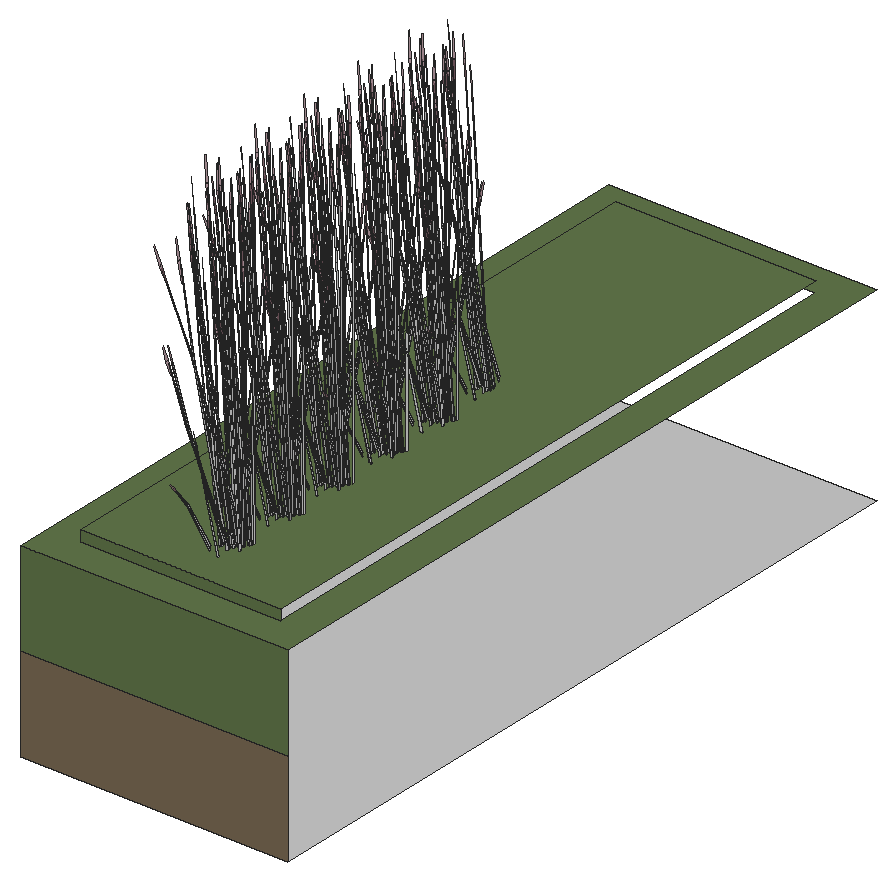
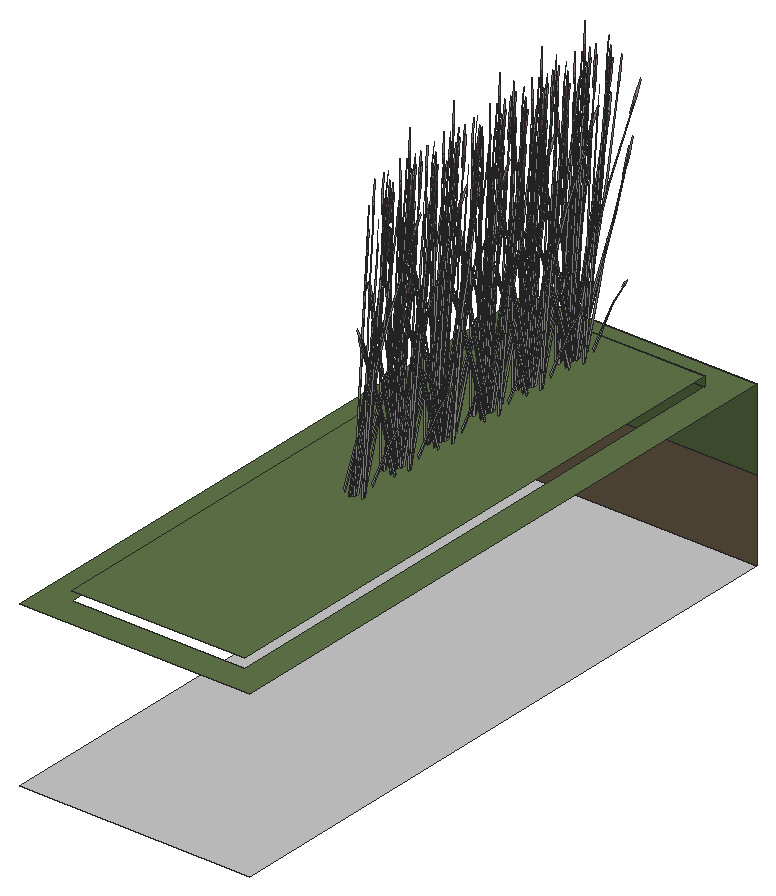
# SketchUp Ruby script. Lengths in inches.
U = 1.inch
M = Sketchup.active_model
def pt(a) = Geom::Point3d.new(a.map { |v| v * U })
def face(e, loops, mat)
  f = e.add_face(loops[0].map { |a| pt(a) })
  loops[1..].each { |l| e.add_face(l.map { |a| pt(a) }).erase! }
  f.material = f.back_material = mat if mat
  f
end
# faces: each face lists its corners as indices into pts; further lists are holes
def faces(e, pts, list, mat = nil) = list.each { |f| face(e, (f[0].is_a?(Array) ? f : [f]).map { |l| l.map { |i| pts[i] } }, mat) }
# xy, xz, yz: faces in a plane at the given z, y or x. An outline is a flat list of corners, or four numbers for a rectangle; further outlines are holes
def ring(l) = l.size == 4 ? [[l[0], l[1]], [l[2], l[1]], [l[2], l[3]], [l[0], l[3]]] : l.each_slice(2).to_a
def flat(e, list, mat, &to3) = list.each { |f| face(e, (f[0].is_a?(Array) ? f : [f]).map { |l| ring(l).map { |u, v| to3.(u, v) } }, mat) }
def xy(e, z, list, mat = nil) = flat(e, list, mat) { |x, y| [x, y, z] }
def xz(e, y, list, mat = nil) = flat(e, list, mat) { |x, z| [x, y, z] }
def yz(e, x, list, mat = nil) = flat(e, list, mat) { |y, z| [x, y, z] }
def lines(e, pts, list) = list.each { |a, b| e.add_line(pt(pts[a]), pt(pts[b])) }
# prism: a flat outline (further loops are holes) pulled along v
def prism(e, loops, v, mat = nil)
  f = face(e, loops, mat); d = Geom::Vector3d.new(v.map { |x| x * U })
  f.pushpull(f.normal.samedirection?(d) ? d.length : -d.length)
end
def box(e, o, s, mat = nil) = prism(e, [[o, [o[0] + s[0], o[1], o[2]], [o[0] + s[0], o[1] + s[1], o[2]], [o[0], o[1] + s[1], o[2]]]], [0, 0, s[2]], mat)
def at(x, y, z, deg = 0) = Geom::Transformation.translation(pt([x, y, z])) * Geom::Transformation.rotation(ORIGIN, Z_AXIS, deg.degrees)
def axes(o, x, y, z) = Geom::Transformation.new([*x, 0, *y, 0, *z, 0, *pt(o).to_a, 1])
def part(name) = M.definitions.add(name)
# library, detail: a bought-in or finely detailed component or shape, given as its bounding box
def library(name, o, s) = part(name).tap { |d| box(d.entities, o, s) }
def detail(e, o, s) = box(e.add_group.entities, o, s)
def put(e, d, t, mat = nil) = e.add_instance(d, t).tap { |i| i.material = mat if mat }
def group(e, t, mat = nil) = e.add_group.tap { |g| g.transformation = t; g.material = mat if mat }.entities
root = M.entities
M.materials.add("LightPink_Translucent").color = [144, 107, 117]
M.materials["LightPink_Translucent"].alpha = 0.75
M.materials.add("Plaster_03_1K").color = [121, 105, 83]
M.materials.add("Roofing_02_1K").color = [97, 118, 74]
M.materials.add("[_0053_Ivory_]").color = [200, 200, 200]
c1 = part("blade")
p = [[2.15,0.21,22],[0,0.17,0],[0.09,0.45,0],[2.18,0.31,22],[2.29,0.31,22],[0.38,0.45,0],
  [2.48,0.24,33],[2.49,0.24,33],[2.48,0.22,33]]
faces(c1.entities,p,[[0,1,2,3],[4,5,2,3],[6,3,4,7],[8,0,3,6]])
c2 = part("seeds")
p = [[0.3,-0.1,1.38],[-0.01,-0.03,1.59],[-0.01,-0.03,0.03],[0.14,-0.07,-0.07],[0.29,-0.03,3],[0.15,0.01,3.11]]
faces(c2.entities,p,[[0,1,2,3],[1,0,4,5]],"LightPink_Translucent")
c3 = part("blade with seeds")
put(c3.entities,c1,at(0,0,0))
put(c3.entities,c2,axes([2.4,0.25,30.99],[1.5799,-0.05474,1.17369],[-0.12525,1.92788,0.29478],[-0.07173,-0.02425,1.56792]))
xy(root,0,[[653.51,239.15,701.51,371.15]],"[_0053_Ivory_]")
xy(root,34,[[[653.51,239.15,701.51,371.15],[659.51,245.15,695.51,365.15]]],"Roofing_02_1K")
xy(root,36,[[659.51,245.15,695.51,365.15]],"Roofing_02_1K")
xz(root,239.15,[[653.51,0,701.51,17]],"Plaster_03_1K")
xz(root,239.15,[[653.51,17,701.51,34]],"Roofing_02_1K")
xz(root,245.15,[[659.51,34,695.51,36]],"Roofing_02_1K")
put(root,c3,axes([677.97,256.68,38.18],[-0.41095,0.33109,-0.35414],[-0.38901,-0.37805,0.4572],[-0.05919,0.19208,0.87481]),"[_0053_Ivory_]")
put(root,c3,axes([677.97,267.83,38.18],[-0.41095,0.33109,-0.35414],[-0.38901,-0.37805,0.4572],[-0.05919,0.19208,0.87481]),"[_0053_Ivory_]")
put(root,c3,axes([677.97,278.82,38.18],[-0.41095,0.33109,-0.35414],[-0.38901,-0.37805,0.4572],[-0.05919,0.19208,0.87481]),"[_0053_Ivory_]")
put(root,c3,axes([677.97,290.87,38.18],[-0.41095,0.33109,-0.35414],[-0.38901,-0.37805,0.4572],[-0.05919,0.19208,0.87481]),"[_0053_Ivory_]")
put(root,c3,axes([677.97,302.23,38.18],[-0.41095,0.33109,-0.35414],[-0.38901,-0.37805,0.4572],[-0.05919,0.19208,0.87481]),"[_0053_Ivory_]")
put(root,c3,axes([680.08,255.69,35.71],[-0.40909,0.47266,-0.62353],[-0.50819,-0.4286,-0.16365],[-0.16393,0.11791,1.37633]),"[_0053_Ivory_]")
put(root,c3,axes([680.08,266.84,35.71],[-0.40909,0.47266,-0.62353],[-0.50819,-0.4286,-0.16365],[-0.16393,0.11791,1.37633]),"[_0053_Ivory_]")
put(root,c3,axes([680.08,277.83,35.71],[-0.40909,0.47266,-0.62353],[-0.50819,-0.4286,-0.16365],[-0.16393,0.11791,1.37633]),"[_0053_Ivory_]")
put(root,c3,axes([680.08,289.875,35.71],[-0.40909,0.47266,-0.62353],[-0.50819,-0.4286,-0.16365],[-0.16393,0.11791,1.37633]),"[_0053_Ivory_]")
put(root,c3,axes([680.08,301.24,35.71],[-0.40909,0.47266,-0.62353],[-0.50819,-0.4286,-0.16365],[-0.16393,0.11791,1.37633]),"[_0053_Ivory_]")
put(root,c3,axes([677.8,254.14,35.98],[-0.56493,0.5287,0.30756],[-0.56528,-0.52313,-0.36492],[-0.01973,-0.15014,1.64885]),"[_0053_Ivory_]")
put(root,c3,axes([677.8,265.29,35.98],[-0.56493,0.5287,0.30756],[-0.56528,-0.52313,-0.36492],[-0.01973,-0.15014,1.64885]),"[_0053_Ivory_]")
put(root,c3,axes([677.8,276.28,35.98],[-0.56493,0.5287,0.30756],[-0.56528,-0.52313,-0.36492],[-0.01973,-0.15014,1.64885]),"[_0053_Ivory_]")
put(root,c3,axes([677.8,288.32,35.98],[-0.56493,0.5287,0.30756],[-0.56528,-0.52313,-0.36492],[-0.01973,-0.15014,1.64885]),"[_0053_Ivory_]")
put(root,c3,axes([677.8,299.69,35.98],[-0.56493,0.5287,0.30756],[-0.56528,-0.52313,-0.36492],[-0.01973,-0.15014,1.64885]),"[_0053_Ivory_]")
put(root,c3,axes([677.8,311.67,35.98],[-0.56493,0.5287,0.30756],[-0.56528,-0.52313,-0.36492],[-0.01973,-0.15014,1.64885]),"[_0053_Ivory_]")
put(root,c3,axes([680.13,255.6,36.98],[0.52485,0.25358,1.51261],[-0.51417,0.54629,0.59816],[-0.23031,-0.32378,1.26806]),"[_0053_Ivory_]")
put(root,c3,axes([680.13,266.75,36.98],[0.52485,0.25358,1.51261],[-0.51417,0.54629,0.59816],[-0.23031,-0.32378,1.26806]),"[_0053_Ivory_]")
put(root,c3,axes([680.13,277.74,36.98],[0.52485,0.25358,1.51261],[-0.51417,0.54629,0.59816],[-0.23031,-0.32378,1.26806]),"[_0053_Ivory_]")
put(root,c3,axes([680.13,289.78,36.98],[0.52485,0.25358,1.51261],[-0.51417,0.54629,0.59816],[-0.23031,-0.32378,1.26806]),"[_0053_Ivory_]")
put(root,c3,axes([680.13,301.15,36.98],[0.52485,0.25358,1.51261],[-0.51417,0.54629,0.59816],[-0.23031,-0.32378,1.26806]),"[_0053_Ivory_]")
put(root,c3,axes([680.13,313.13,36.98],[0.52485,0.25358,1.51261],[-0.51417,0.54629,0.59816],[-0.23031,-0.32378,1.26806]),"[_0053_Ivory_]")
put(root,c3,axes([678.125,251,36.42],[0.31682,0.21887,1.1486],[-0.4614,0.13157,0.84392],[-0.09872,-0.16821,0.25299]),"[_0053_Ivory_]")
put(root,c3,axes([678.125,262.15,36.42],[0.31682,0.21887,1.1486],[-0.4614,0.13157,0.84392],[-0.09872,-0.16821,0.25299]),"[_0053_Ivory_]")
put(root,c3,axes([678.125,273.14,36.42],[0.31682,0.21887,1.1486],[-0.4614,0.13157,0.84392],[-0.09872,-0.16821,0.25299]),"[_0053_Ivory_]")
put(root,c3,axes([678.125,285.18,36.42],[0.31682,0.21887,1.1486],[-0.4614,0.13157,0.84392],[-0.09872,-0.16821,0.25299]),"[_0053_Ivory_]")
put(root,c3,axes([678.125,296.55,36.42],[0.31682,0.21887,1.1486],[-0.4614,0.13157,0.84392],[-0.09872,-0.16821,0.25299]),"[_0053_Ivory_]")
put(root,c3,axes([678.125,308.53,36.42],[0.31682,0.21887,1.1486],[-0.4614,0.13157,0.84392],[-0.09872,-0.16821,0.25299]),"[_0053_Ivory_]")
put(root,c3,axes([680.36,255.43,36.12],[-0.59306,-0.50614,-0.25192],[0.49904,-0.56836,0.5513],[-0.1597,0.05921,1.68216]),"[_0053_Ivory_]")
put(root,c3,axes([680.36,266.57,36.12],[-0.59306,-0.50614,-0.25192],[0.49904,-0.56836,0.5513],[-0.1597,0.05921,1.68216]),"[_0053_Ivory_]")
put(root,c3,axes([680.36,277.57,36.12],[-0.59306,-0.50614,-0.25192],[0.49904,-0.56836,0.5513],[-0.1597,0.05921,1.68216]),"[_0053_Ivory_]")
put(root,c3,axes([680.36,289.61,36.12],[-0.59306,-0.50614,-0.25192],[0.49904,-0.56836,0.5513],[-0.1597,0.05921,1.68216]),"[_0053_Ivory_]")
put(root,c3,axes([680.36,300.98,36.12],[-0.59306,-0.50614,-0.25192],[0.49904,-0.56836,0.5513],[-0.1597,0.05921,1.68216]),"[_0053_Ivory_]")
put(root,c3,axes([679.28,254.9375,35.86],[-0.36485,-0.52782,-0.44739],[0.55265,-0.37168,0.21531],[-0.11807,-0.06531,1.43643]),"[_0053_Ivory_]")
put(root,c3,axes([679.28,266.09,35.86],[-0.36485,-0.52782,-0.44739],[0.55265,-0.37168,0.21531],[-0.11807,-0.06531,1.43643]),"[_0053_Ivory_]")
put(root,c3,axes([679.28,277.08,35.86],[-0.36485,-0.52782,-0.44739],[0.55265,-0.37168,0.21531],[-0.11807,-0.06531,1.43643]),"[_0053_Ivory_]")
put(root,c3,axes([679.28,289.12,35.86],[-0.36485,-0.52782,-0.44739],[0.55265,-0.37168,0.21531],[-0.11807,-0.06531,1.43643]),"[_0053_Ivory_]")
put(root,c3,axes([679.28,300.49,35.86],[-0.36485,-0.52782,-0.44739],[0.55265,-0.37168,0.21531],[-0.11807,-0.06531,1.43643]),"[_0053_Ivory_]")
put(root,c3,axes([679.28,312.47,35.86],[-0.36485,-0.52782,-0.44739],[0.55265,-0.37168,0.21531],[-0.11807,-0.06531,1.43643]),"[_0053_Ivory_]")
put(root,c3,axes([678.25,256.33,38.99],[-0.0158,0.58168,-0.7886],[-0.66548,-0.03907,0.09517],[-0.07023,0.24643,1.11556]),"[_0053_Ivory_]")
put(root,c3,axes([678.25,267.48,38.99],[-0.0158,0.58168,-0.7886],[-0.66548,-0.03907,0.09517],[-0.07023,0.24643,1.11556]),"[_0053_Ivory_]")
put(root,c3,axes([678.25,278.47,38.99],[-0.0158,0.58168,-0.7886],[-0.66548,-0.03907,0.09517],[-0.07023,0.24643,1.11556]),"[_0053_Ivory_]")
put(root,c3,axes([678.25,290.52,38.99],[-0.0158,0.58168,-0.7886],[-0.66548,-0.03907,0.09517],[-0.07023,0.24643,1.11556]),"[_0053_Ivory_]")
put(root,c3,axes([678.25,301.88,38.99],[-0.0158,0.58168,-0.7886],[-0.66548,-0.03907,0.09517],[-0.07023,0.24643,1.11556]),"[_0053_Ivory_]")
put(root,c3,axes([678.24,257.97,36.42],[-0.01572,-0.37392,1.1486],[0.39276,0.26669,0.84392],[-0.07724,0.17822,0.25299]),"[_0053_Ivory_]")
put(root,c3,axes([678.24,269.12,36.42],[-0.01572,-0.37392,1.1486],[0.39276,0.26669,0.84392],[-0.07724,0.17822,0.25299]),"[_0053_Ivory_]")
put(root,c3,axes([678.24,280.11,36.42],[-0.01572,-0.37392,1.1486],[0.39276,0.26669,0.84392],[-0.07724,0.17822,0.25299]),"[_0053_Ivory_]")
put(root,c3,axes([678.24,292.15,36.42],[-0.01572,-0.37392,1.1486],[0.39276,0.26669,0.84392],[-0.07724,0.17822,0.25299]),"[_0053_Ivory_]")
put(root,c3,axes([678.24,303.52,36.42],[-0.01572,-0.37392,1.1486],[0.39276,0.26669,0.84392],[-0.07724,0.17822,0.25299]),"[_0053_Ivory_]")
put(root,c3,axes([680.06,255.32,35.86],[-0.65953,0.03882,-0.44739],[-0.05964,-0.64439,0.21531],[-0.11807,0.06531,1.43643]),"[_0053_Ivory_]")
put(root,c3,axes([680.06,266.47,35.86],[-0.65953,0.03882,-0.44739],[-0.05964,-0.64439,0.21531],[-0.11807,0.06531,1.43643]),"[_0053_Ivory_]")
put(root,c3,axes([680.06,277.46,35.86],[-0.65953,0.03882,-0.44739],[-0.05964,-0.64439,0.21531],[-0.11807,0.06531,1.43643]),"[_0053_Ivory_]")
put(root,c3,axes([680.06,289.5,35.86],[-0.65953,0.03882,-0.44739],[-0.05964,-0.64439,0.21531],[-0.11807,0.06531,1.43643]),"[_0053_Ivory_]")
put(root,c3,axes([680.06,300.87,35.86],[-0.65953,0.03882,-0.44739],[-0.05964,-0.64439,0.21531],[-0.11807,0.06531,1.43643]),"[_0053_Ivory_]")
put(root,c3,axes([678.8,256.4,36.13],[0.56842,0.31443,0.49651],[-0.33976,0.56381,0],[-0.12946,-0.07161,1.57504]),"[_0053_Ivory_]")
put(root,c3,axes([678.8,267.54,36.13],[0.56842,0.31443,0.49651],[-0.33976,0.56381,0],[-0.12946,-0.07161,1.57504]),"[_0053_Ivory_]")
put(root,c3,axes([678.8,278.54,36.13],[0.56842,0.31443,0.49651],[-0.33976,0.56381,0],[-0.12946,-0.07161,1.57504]),"[_0053_Ivory_]")
put(root,c3,axes([678.8,290.58,36.13],[0.56842,0.31443,0.49651],[-0.33976,0.56381,0],[-0.12946,-0.07161,1.57504]),"[_0053_Ivory_]")
put(root,c3,axes([678.8,301.95,36.13],[0.56842,0.31443,0.49651],[-0.33976,0.56381,0],[-0.12946,-0.07161,1.57504]),"[_0053_Ivory_]")
put(root,c3,axes([678.03,257.15,37.02],[0.01334,-0.32463,1.54345],[0.60018,0.17147,0.21329],[-0.052,0.34598,0.72882]),"[_0053_Ivory_]")
put(root,c3,axes([678.03,268.3,37.02],[0.01334,-0.32463,1.54345],[0.60018,0.17147,0.21329],[-0.052,0.34598,0.72882]),"[_0053_Ivory_]")
put(root,c3,axes([678.03,279.29,37.02],[0.01334,-0.32463,1.54345],[0.60018,0.17147,0.21329],[-0.052,0.34598,0.72882]),"[_0053_Ivory_]")
put(root,c3,axes([678.03,291.33,37.02],[0.01334,-0.32463,1.54345],[0.60018,0.17147,0.21329],[-0.052,0.34598,0.72882]),"[_0053_Ivory_]")
put(root,c3,axes([678.03,302.7,37.02],[0.01334,-0.32463,1.54345],[0.60018,0.17147,0.21329],[-0.052,0.34598,0.72882]),"[_0053_Ivory_]")
put(root,c3,axes([679.33,255.24,36.09],[0.16098,-0.74515,-0.23429],[0.76326,0.12989,0.51271],[-0.13337,-0.1029,1.5644]),"[_0053_Ivory_]")
put(root,c3,axes([679.33,266.39,36.09],[0.16098,-0.74515,-0.23429],[0.76326,0.12989,0.51271],[-0.13337,-0.1029,1.5644]),"[_0053_Ivory_]")
put(root,c3,axes([679.33,277.38,36.09],[0.16098,-0.74515,-0.23429],[0.76326,0.12989,0.51271],[-0.13337,-0.1029,1.5644]),"[_0053_Ivory_]")
put(root,c3,axes([679.33,289.42,36.09],[0.16098,-0.74515,-0.23429],[0.76326,0.12989,0.51271],[-0.13337,-0.1029,1.5644]),"[_0053_Ivory_]")
put(root,c3,axes([679.33,300.79,36.09],[0.16098,-0.74515,-0.23429],[0.76326,0.12989,0.51271],[-0.13337,-0.1029,1.5644]),"[_0053_Ivory_]")
put(root,c3,axes([679.33,312.77,36.09],[0.16098,-0.74515,-0.23429],[0.76326,0.12989,0.51271],[-0.13337,-0.1029,1.5644]),"[_0053_Ivory_]")
put(root,c3,axes([679.61,255.42,36.27],[-0.11717,0.56122,0.1448],[-0.57245,-0.09742,-0.41347],[-0.10418,-0.05763,1.26744]),"[_0053_Ivory_]")
put(root,c3,axes([679.61,266.57,36.27],[-0.11717,0.56122,0.1448],[-0.57245,-0.09742,-0.41347],[-0.10418,-0.05763,1.26744]),"[_0053_Ivory_]")
put(root,c3,axes([679.61,277.56,36.27],[-0.11717,0.56122,0.1448],[-0.57245,-0.09742,-0.41347],[-0.10418,-0.05763,1.26744]),"[_0053_Ivory_]")
put(root,c3,axes([679.61,289.6,36.27],[-0.11717,0.56122,0.1448],[-0.57245,-0.09742,-0.41347],[-0.10418,-0.05763,1.26744]),"[_0053_Ivory_]")
put(root,c3,axes([679.61,300.97,36.27],[-0.11717,0.56122,0.1448],[-0.57245,-0.09742,-0.41347],[-0.10418,-0.05763,1.26744]),"[_0053_Ivory_]")
put(root,c3,axes([680.75,256.98,35.67],[-0.56842,0.31443,-0.49651],[-0.33976,-0.56381,0],[-0.12946,0.07161,1.57504]),"[_0053_Ivory_]")
put(root,c3,axes([680.75,268.13,35.67],[-0.56842,0.31443,-0.49651],[-0.33976,-0.56381,0],[-0.12946,0.07161,1.57504]),"[_0053_Ivory_]")
put(root,c3,axes([680.75,279.12,35.67],[-0.56842,0.31443,-0.49651],[-0.33976,-0.56381,0],[-0.12946,0.07161,1.57504]),"[_0053_Ivory_]")
put(root,c3,axes([680.75,291.16,35.67],[-0.56842,0.31443,-0.49651],[-0.33976,-0.56381,0],[-0.12946,0.07161,1.57504]),"[_0053_Ivory_]")
put(root,c3,axes([680.75,302.53,35.67],[-0.56842,0.31443,-0.49651],[-0.33976,-0.56381,0],[-0.12946,0.07161,1.57504]),"[_0053_Ivory_]")
put(root,c3,axes([677.39,253.85,35.67],[0,-0.62885,-0.49651],[0.67951,0,0],[0,-0.14322,1.57504]),"[_0053_Ivory_]")
put(root,c3,axes([677.39,265,35.67],[0,-0.62885,-0.49651],[0.67951,0,0],[0,-0.14322,1.57504]),"[_0053_Ivory_]")
put(root,c3,axes([677.39,275.99,35.67],[0,-0.62885,-0.49651],[0.67951,0,0],[0,-0.14322,1.57504]),"[_0053_Ivory_]")
put(root,c3,axes([677.39,288.03,35.67],[0,-0.62885,-0.49651],[0.67951,0,0],[0,-0.14322,1.57504]),"[_0053_Ivory_]")
put(root,c3,axes([677.39,299.4,35.67],[0,-0.62885,-0.49651],[0.67951,0,0],[0,-0.14322,1.57504]),"[_0053_Ivory_]")
put(root,c3,axes([677.39,311.375,35.67],[0,-0.62885,-0.49651],[0.67951,0,0],[0,-0.14322,1.57504]),"[_0053_Ivory_]")
put(root,c3,axes([677.68,254.43,36.13],[0,0.62885,0.49651],[-0.67951,0,0],[0,-0.14322,1.57504]),"[_0053_Ivory_]")
put(root,c3,axes([677.68,265.58,36.13],[0,0.62885,0.49651],[-0.67951,0,0],[0,-0.14322,1.57504]),"[_0053_Ivory_]")
put(root,c3,axes([677.68,276.57,36.13],[0,0.62885,0.49651],[-0.67951,0,0],[0,-0.14322,1.57504]),"[_0053_Ivory_]")
put(root,c3,axes([677.68,288.61,36.13],[0,0.62885,0.49651],[-0.67951,0,0],[0,-0.14322,1.57504]),"[_0053_Ivory_]")
put(root,c3,axes([677.68,299.98,36.13],[0,0.62885,0.49651],[-0.67951,0,0],[0,-0.14322,1.57504]),"[_0053_Ivory_]")
put(root,c3,axes([677.68,311.96,36.13],[0,0.62885,0.49651],[-0.67951,0,0],[0,-0.14322,1.57504]),"[_0053_Ivory_]")
put(root,c3,axes([680.79,256.8125,35.85],[-0.37499,-0.63235,-0.05142],[0.6353,-0.35142,0.51607],[-0.15655,0.0602,1.6363]),"[_0053_Ivory_]")
put(root,c3,axes([680.79,267.96,35.85],[-0.37499,-0.63235,-0.05142],[0.6353,-0.35142,0.51607],[-0.15655,0.0602,1.6363]),"[_0053_Ivory_]")
put(root,c3,axes([680.79,278.95,35.85],[-0.37499,-0.63235,-0.05142],[0.6353,-0.35142,0.51607],[-0.15655,0.0602,1.6363]),"[_0053_Ivory_]")
put(root,c3,axes([680.79,291,35.85],[-0.37499,-0.63235,-0.05142],[0.6353,-0.35142,0.51607],[-0.15655,0.0602,1.6363]),"[_0053_Ivory_]")
put(root,c3,axes([680.79,302.36,35.85],[-0.37499,-0.63235,-0.05142],[0.6353,-0.35142,0.51607],[-0.15655,0.0602,1.6363]),"[_0053_Ivory_]")
put(root,c3,axes([678.38,256.53,38.66],[0.43478,0.42253,-0.5672],[-0.45929,0.37004,-0.43934],[-0.06615,0.21468,1.08528]),"[_0053_Ivory_]")
put(root,c3,axes([678.38,267.67,38.66],[0.43478,0.42253,-0.5672],[-0.45929,0.37004,-0.43934],[-0.06615,0.21468,1.08528]),"[_0053_Ivory_]")
put(root,c3,axes([678.38,278.67,38.66],[0.43478,0.42253,-0.5672],[-0.45929,0.37004,-0.43934],[-0.06615,0.21468,1.08528]),"[_0053_Ivory_]")
put(root,c3,axes([678.38,290.71,38.66],[0.43478,0.42253,-0.5672],[-0.45929,0.37004,-0.43934],[-0.06615,0.21468,1.08528]),"[_0053_Ivory_]")
put(root,c3,axes([678.38,302.08,38.66],[0.43478,0.42253,-0.5672],[-0.45929,0.37004,-0.43934],[-0.06615,0.21468,1.08528]),"[_0053_Ivory_]")
put(root,c3,axes([680.62,256.73,35.68],[-0.56663,-0.1556,-0.30978],[0.14267,-0.54795,0.30978],[-0.11423,0.06319,1.38974]),"[_0053_Ivory_]")
put(root,c3,axes([680.62,267.88,35.68],[-0.56663,-0.1556,-0.30978],[0.14267,-0.54795,0.30978],[-0.11423,0.06319,1.38974]),"[_0053_Ivory_]")
put(root,c3,axes([680.62,278.87,35.68],[-0.56663,-0.1556,-0.30978],[0.14267,-0.54795,0.30978],[-0.11423,0.06319,1.38974]),"[_0053_Ivory_]")
put(root,c3,axes([680.62,290.92,35.68],[-0.56663,-0.1556,-0.30978],[0.14267,-0.54795,0.30978],[-0.11423,0.06319,1.38974]),"[_0053_Ivory_]")
put(root,c3,axes([680.62,302.28,35.68],[-0.56663,-0.1556,-0.30978],[0.14267,-0.54795,0.30978],[-0.11423,0.06319,1.38974]),"[_0053_Ivory_]")
put(root,c3,axes([679.16,254.58,36.32],[-0.68399,-0.30005,-0.29095],[0.32934,-0.63331,-0.50002],[-0.0215,-0.15549,1.59708]),"[_0053_Ivory_]")
put(root,c3,axes([679.16,265.72,36.32],[-0.68399,-0.30005,-0.29095],[0.32934,-0.63331,-0.50002],[-0.0215,-0.15549,1.59708]),"[_0053_Ivory_]")
put(root,c3,axes([679.16,276.72,36.32],[-0.68399,-0.30005,-0.29095],[0.32934,-0.63331,-0.50002],[-0.0215,-0.15549,1.59708]),"[_0053_Ivory_]")
put(root,c3,axes([679.16,288.76,36.32],[-0.68399,-0.30005,-0.29095],[0.32934,-0.63331,-0.50002],[-0.0215,-0.15549,1.59708]),"[_0053_Ivory_]")
put(root,c3,axes([679.16,300.125,36.32],[-0.68399,-0.30005,-0.29095],[0.32934,-0.63331,-0.50002],[-0.0215,-0.15549,1.59708]),"[_0053_Ivory_]")
put(root,c3,axes([679.16,312.1,36.32],[-0.68399,-0.30005,-0.29095],[0.32934,-0.63331,-0.50002],[-0.0215,-0.15549,1.59708]),"[_0053_Ivory_]")
put(root,c3,axes([680.94,254.39,36.5],[-0.01659,-0.59209,1.41272],[0.75089,0.15348,0.59816],[-0.1776,0.32398,1.3335]),"[_0053_Ivory_]")
put(root,c3,axes([680.94,265.54,36.5],[-0.01659,-0.59209,1.41272],[0.75089,0.15348,0.59816],[-0.1776,0.32398,1.3335]),"[_0053_Ivory_]")
put(root,c3,axes([680.94,276.53,36.5],[-0.01659,-0.59209,1.41272],[0.75089,0.15348,0.59816],[-0.1776,0.32398,1.3335]),"[_0053_Ivory_]")
put(root,c3,axes([680.94,288.57,36.5],[-0.01659,-0.59209,1.41272],[0.75089,0.15348,0.59816],[-0.1776,0.32398,1.3335]),"[_0053_Ivory_]")
put(root,c3,axes([680.94,299.94,36.5],[-0.01659,-0.59209,1.41272],[0.75089,0.15348,0.59816],[-0.1776,0.32398,1.3335]),"[_0053_Ivory_]")
put(root,c3,axes([677.91,257.16,36.48],[0.55175,-0.11136,0.06507],[0.12684,0.44864,-0.86304],[-0.03498,0.22711,0.7736]),"[_0053_Ivory_]")
put(root,c3,axes([677.91,268.31,36.48],[0.55175,-0.11136,0.06507],[0.12684,0.44864,-0.86304],[-0.03498,0.22711,0.7736]),"[_0053_Ivory_]")
put(root,c3,axes([677.91,279.3,36.48],[0.55175,-0.11136,0.06507],[0.12684,0.44864,-0.86304],[-0.03498,0.22711,0.7736]),"[_0053_Ivory_]")
put(root,c3,axes([677.91,291.34,36.48],[0.55175,-0.11136,0.06507],[0.12684,0.44864,-0.86304],[-0.03498,0.22711,0.7736]),"[_0053_Ivory_]")
put(root,c3,axes([677.91,302.71,36.48],[0.55175,-0.11136,0.06507],[0.12684,0.44864,-0.86304],[-0.03498,0.22711,0.7736]),"[_0053_Ivory_]")
put(root,c3,axes([680.52,255.14,36.32],[0.07077,0.71755,-0.29095],[-0.73712,0.04339,-0.50002],[-0.1298,0.09558,1.59708]),"[_0053_Ivory_]")
put(root,c3,axes([680.52,266.29,36.32],[0.07077,0.71755,-0.29095],[-0.73712,0.04339,-0.50002],[-0.1298,0.09558,1.59708]),"[_0053_Ivory_]")
put(root,c3,axes([680.52,277.28,36.32],[0.07077,0.71755,-0.29095],[-0.73712,0.04339,-0.50002],[-0.1298,0.09558,1.59708]),"[_0053_Ivory_]")
put(root,c3,axes([680.52,289.33,36.32],[0.07077,0.71755,-0.29095],[-0.73712,0.04339,-0.50002],[-0.1298,0.09558,1.59708]),"[_0053_Ivory_]")
put(root,c3,axes([680.52,300.69,36.32],[0.07077,0.71755,-0.29095],[-0.73712,0.04339,-0.50002],[-0.1298,0.09558,1.59708]),"[_0053_Ivory_]")
put(root,c3,axes([678.86,253.9375,35.75],[-0.24943,-0.64486,-0.69835],[0.71849,-0.23224,-0.18329],[-0.02757,-0.21836,1.54149]),"[_0053_Ivory_]")
put(root,c3,axes([678.86,265.09,35.75],[-0.24943,-0.64486,-0.69835],[0.71849,-0.23224,-0.18329],[-0.02757,-0.21836,1.54149]),"[_0053_Ivory_]")
put(root,c3,axes([678.86,276.08,35.75],[-0.24943,-0.64486,-0.69835],[0.71849,-0.23224,-0.18329],[-0.02757,-0.21836,1.54149]),"[_0053_Ivory_]")
put(root,c3,axes([678.86,288.12,35.75],[-0.24943,-0.64486,-0.69835],[0.71849,-0.23224,-0.18329],[-0.02757,-0.21836,1.54149]),"[_0053_Ivory_]")
put(root,c3,axes([678.86,299.49,35.75],[-0.24943,-0.64486,-0.69835],[0.71849,-0.23224,-0.18329],[-0.02757,-0.21836,1.54149]),"[_0053_Ivory_]")
put(root,c3,axes([678.86,311.47,35.75],[-0.24943,-0.64486,-0.69835],[0.71849,-0.23224,-0.18329],[-0.02757,-0.21836,1.54149]),"[_0053_Ivory_]")
put(root,c3,axes([679.98,251.91,38.33],[-0.59704,-0.15764,-0.51099],[0.20464,-0.54049,-0.3958],[-0.05475,-0.21761,0.97773]),"[_0053_Ivory_]")
put(root,c3,axes([679.98,263.0625,38.33],[-0.59704,-0.15764,-0.51099],[0.20464,-0.54049,-0.3958],[-0.05475,-0.21761,0.97773]),"[_0053_Ivory_]")
put(root,c3,axes([679.98,274.05,38.33],[-0.59704,-0.15764,-0.51099],[0.20464,-0.54049,-0.3958],[-0.05475,-0.21761,0.97773]),"[_0053_Ivory_]")
put(root,c3,axes([679.98,286.1,38.33],[-0.59704,-0.15764,-0.51099],[0.20464,-0.54049,-0.3958],[-0.05475,-0.21761,0.97773]),"[_0053_Ivory_]")
put(root,c3,axes([679.98,297.47,38.33],[-0.59704,-0.15764,-0.51099],[0.20464,-0.54049,-0.3958],[-0.05475,-0.21761,0.97773]),"[_0053_Ivory_]")
put(root,c3,axes([679.98,309.44,38.33],[-0.59704,-0.15764,-0.51099],[0.20464,-0.54049,-0.3958],[-0.05475,-0.21761,0.97773]),"[_0053_Ivory_]")
put(root,c3,axes([678.88,255.92,37.53],[-0.01487,-0.24136,1.71376],[0.64429,0.16012,0.13857],[-0.03985,0.34396,0.73262]),"[_0053_Ivory_]")
put(root,c3,axes([678.88,267.07,37.53],[-0.01487,-0.24136,1.71376],[0.64429,0.16012,0.13857],[-0.03985,0.34396,0.73262]),"[_0053_Ivory_]")
put(root,c3,axes([678.88,278.06,37.53],[-0.01487,-0.24136,1.71376],[0.64429,0.16012,0.13857],[-0.03985,0.34396,0.73262]),"[_0053_Ivory_]")
put(root,c3,axes([678.88,290.1,37.53],[-0.01487,-0.24136,1.71376],[0.64429,0.16012,0.13857],[-0.03985,0.34396,0.73262]),"[_0053_Ivory_]")
put(root,c3,axes([678.88,301.47,37.53],[-0.01487,-0.24136,1.71376],[0.64429,0.16012,0.13857],[-0.03985,0.34396,0.73262]),"[_0053_Ivory_]")
put(root,c3,axes([677.68,253.86,35.68],[0.42396,-0.39235,-0.30978],[0.42396,0.39235,0.30978],[0,-0.12637,1.38974]),"[_0053_Ivory_]")
put(root,c3,axes([677.68,265.01,35.68],[0.42396,-0.39235,-0.30978],[0.42396,0.39235,0.30978],[0,-0.12637,1.38974]),"[_0053_Ivory_]")
put(root,c3,axes([677.68,276,35.68],[0.42396,-0.39235,-0.30978],[0.42396,0.39235,0.30978],[0,-0.12637,1.38974]),"[_0053_Ivory_]")
put(root,c3,axes([677.68,288.04,35.68],[0.42396,-0.39235,-0.30978],[0.42396,0.39235,0.30978],[0,-0.12637,1.38974]),"[_0053_Ivory_]")
put(root,c3,axes([677.68,299.41,35.68],[0.42396,-0.39235,-0.30978],[0.42396,0.39235,0.30978],[0,-0.12637,1.38974]),"[_0053_Ivory_]")
put(root,c3,axes([677.68,311.39,35.68],[0.42396,-0.39235,-0.30978],[0.42396,0.39235,0.30978],[0,-0.12637,1.38974]),"[_0053_Ivory_]")
put(root,c3,axes([679.59,251.32,35.78],[-0.4197,0.36076,-0.03893],[-0.38456,-0.39511,-0.17649],[-0.02707,-0.11196,0.58215]),"[_0053_Ivory_]")
put(root,c3,axes([679.59,262.47,35.78],[-0.4197,0.36076,-0.03893],[-0.38456,-0.39511,-0.17649],[-0.02707,-0.11196,0.58215]),"[_0053_Ivory_]")
put(root,c3,axes([679.59,273.46,35.78],[-0.4197,0.36076,-0.03893],[-0.38456,-0.39511,-0.17649],[-0.02707,-0.11196,0.58215]),"[_0053_Ivory_]")
put(root,c3,axes([679.59,285.51,35.78],[-0.4197,0.36076,-0.03893],[-0.38456,-0.39511,-0.17649],[-0.02707,-0.11196,0.58215]),"[_0053_Ivory_]")
put(root,c3,axes([679.59,296.875,35.78],[-0.4197,0.36076,-0.03893],[-0.38456,-0.39511,-0.17649],[-0.02707,-0.11196,0.58215]),"[_0053_Ivory_]")
put(root,c3,axes([679.59,308.85,35.78],[-0.4197,0.36076,-0.03893],[-0.38456,-0.39511,-0.17649],[-0.02707,-0.11196,0.58215]),"[_0053_Ivory_]")
put(root,c3,axes([679.42,254.88,36.01],[0.76764,0.13249,0.45755],[-0.15622,0.74829,0.17955],[-0.11218,-0.07226,1.58856]),"[_0053_Ivory_]")
put(root,c3,axes([679.42,266.03,36.01],[0.76764,0.13249,0.45755],[-0.15622,0.74829,0.17955],[-0.11218,-0.07226,1.58856]),"[_0053_Ivory_]")
put(root,c3,axes([679.42,277.02,36.01],[0.76764,0.13249,0.45755],[-0.15622,0.74829,0.17955],[-0.11218,-0.07226,1.58856]),"[_0053_Ivory_]")
put(root,c3,axes([679.42,289.07,36.01],[0.76764,0.13249,0.45755],[-0.15622,0.74829,0.17955],[-0.11218,-0.07226,1.58856]),"[_0053_Ivory_]")
put(root,c3,axes([679.42,300.43,36.01],[0.76764,0.13249,0.45755],[-0.15622,0.74829,0.17955],[-0.11218,-0.07226,1.58856]),"[_0053_Ivory_]")
put(root,c3,axes([679.22,254.75,36.37],[-0.29468,0.56664,0.44739],[-0.61229,-0.27271,-0.21531],[0,-0.13062,1.43643]),"[_0053_Ivory_]")
put(root,c3,axes([679.22,265.9,36.37],[-0.29468,0.56664,0.44739],[-0.61229,-0.27271,-0.21531],[0,-0.13062,1.43643]),"[_0053_Ivory_]")
put(root,c3,axes([679.22,276.89,36.37],[-0.29468,0.56664,0.44739],[-0.61229,-0.27271,-0.21531],[0,-0.13062,1.43643]),"[_0053_Ivory_]")
put(root,c3,axes([679.22,288.93,36.37],[-0.29468,0.56664,0.44739],[-0.61229,-0.27271,-0.21531],[0,-0.13062,1.43643]),"[_0053_Ivory_]")
put(root,c3,axes([679.22,300.3,36.37],[-0.29468,0.56664,0.44739],[-0.61229,-0.27271,-0.21531],[0,-0.13062,1.43643]),"[_0053_Ivory_]")
put(root,c3,axes([679.22,312.28,36.37],[-0.29468,0.56664,0.44739],[-0.61229,-0.27271,-0.21531],[0,-0.13062,1.43643]),"[_0053_Ivory_]")
put(root,c3,axes([680.2,252.02,38.63],[-0.28988,-0.51132,-0.71045],[0.59671,-0.28496,0.08574],[-0.06778,-0.24706,1.00501]),"[_0053_Ivory_]")
put(root,c3,axes([680.2,263.17,38.63],[-0.28988,-0.51132,-0.71045],[0.59671,-0.28496,0.08574],[-0.06778,-0.24706,1.00501]),"[_0053_Ivory_]")
put(root,c3,axes([680.2,274.16,38.63],[-0.28988,-0.51132,-0.71045],[0.59671,-0.28496,0.08574],[-0.06778,-0.24706,1.00501]),"[_0053_Ivory_]")
put(root,c3,axes([680.2,286.2,38.63],[-0.28988,-0.51132,-0.71045],[0.59671,-0.28496,0.08574],[-0.06778,-0.24706,1.00501]),"[_0053_Ivory_]")
put(root,c3,axes([680.2,297.57,38.63],[-0.28988,-0.51132,-0.71045],[0.59671,-0.28496,0.08574],[-0.06778,-0.24706,1.00501]),"[_0053_Ivory_]")
put(root,c3,axes([680.2,309.55,38.63],[-0.28988,-0.51132,-0.71045],[0.59671,-0.28496,0.08574],[-0.06778,-0.24706,1.00501]),"[_0053_Ivory_]")
put(root,c3,axes([679.01,256.08,36.13],[0.65264,-0.16691,0.17642],[0.16115,0.62115,0.35086],[-0.05821,-0.0905,1.60407]),"[_0053_Ivory_]")
put(root,c3,axes([679.01,267.23,36.13],[0.65264,-0.16691,0.17642],[0.16115,0.62115,0.35086],[-0.05821,-0.0905,1.60407]),"[_0053_Ivory_]")
put(root,c3,axes([679.01,278.22,36.13],[0.65264,-0.16691,0.17642],[0.16115,0.62115,0.35086],[-0.05821,-0.0905,1.60407]),"[_0053_Ivory_]")
put(root,c3,axes([679.01,290.26,36.13],[0.65264,-0.16691,0.17642],[0.16115,0.62115,0.35086],[-0.05821,-0.0905,1.60407]),"[_0053_Ivory_]")
put(root,c3,axes([679.01,301.63,36.13],[0.65264,-0.16691,0.17642],[0.16115,0.62115,0.35086],[-0.05821,-0.0905,1.60407]),"[_0053_Ivory_]")
put(root,c3,axes([679.85,256.18,35.85],[-0.61229,-0.28233,0],[0.29468,-0.58663,0],[0,0,1.62707]),"[_0053_Ivory_]")
put(root,c3,axes([679.85,267.33,35.85],[-0.61229,-0.28233,0],[0.29468,-0.58663,0],[0,0,1.62707]),"[_0053_Ivory_]")
put(root,c3,axes([679.85,278.32,35.85],[-0.61229,-0.28233,0],[0.29468,-0.58663,0],[0,0,1.62707]),"[_0053_Ivory_]")
put(root,c3,axes([679.85,290.36,35.85],[-0.61229,-0.28233,0],[0.29468,-0.58663,0],[0,0,1.62707]),"[_0053_Ivory_]")
put(root,c3,axes([679.85,301.73,35.85],[-0.61229,-0.28233,0],[0.29468,-0.58663,0],[0,0,1.62707]),"[_0053_Ivory_]")
put(root,c3,axes([681.27,256.88,36.03],[0.37973,0.63014,0],[-0.6353,0.35142,-0.51607],[-0.14469,0.08004,1.63711]),"[_0053_Ivory_]")
put(root,c3,axes([681.27,268.03,36.03],[0.37973,0.63014,0],[-0.6353,0.35142,-0.51607],[-0.14469,0.08004,1.63711]),"[_0053_Ivory_]")
put(root,c3,axes([681.27,279.02,36.03],[0.37973,0.63014,0],[-0.6353,0.35142,-0.51607],[-0.14469,0.08004,1.63711]),"[_0053_Ivory_]")
put(root,c3,axes([681.27,291.07,36.03],[0.37973,0.63014,0],[-0.6353,0.35142,-0.51607],[-0.14469,0.08004,1.63711]),"[_0053_Ivory_]")
put(root,c3,axes([681.27,302.43,36.03],[0.37973,0.63014,0],[-0.6353,0.35142,-0.51607],[-0.14469,0.08004,1.63711]),"[_0053_Ivory_]")
put(root,c3,axes([680.95,256.11,36.13],[0.17545,-0.62497,0.17642],[0.64204,0.17686,0.35086],[-0.11091,0.00304,1.60407]),"[_0053_Ivory_]")
put(root,c3,axes([680.95,267.26,36.13],[0.17545,-0.62497,0.17642],[0.64204,0.17686,0.35086],[-0.11091,0.00304,1.60407]),"[_0053_Ivory_]")
put(root,c3,axes([680.95,278.25,36.13],[0.17545,-0.62497,0.17642],[0.64204,0.17686,0.35086],[-0.11091,0.00304,1.60407]),"[_0053_Ivory_]")
put(root,c3,axes([680.95,290.3,36.13],[0.17545,-0.62497,0.17642],[0.64204,0.17686,0.35086],[-0.11091,0.00304,1.60407]),"[_0053_Ivory_]")
put(root,c3,axes([680.95,301.66,36.13],[0.17545,-0.62497,0.17642],[0.64204,0.17686,0.35086],[-0.11091,0.00304,1.60407]),"[_0053_Ivory_]")
put(root,c3,axes([680.66,255.28,36.27],[0.44871,0.37783,0.1448],[-0.37428,0.42627,-0.41347],[-0.10418,0.05763,1.26744]),"[_0053_Ivory_]")
put(root,c3,axes([680.66,266.43,36.27],[0.44871,0.37783,0.1448],[-0.37428,0.42627,-0.41347],[-0.10418,0.05763,1.26744]),"[_0053_Ivory_]")
put(root,c3,axes([680.66,277.42,36.27],[0.44871,0.37783,0.1448],[-0.37428,0.42627,-0.41347],[-0.10418,0.05763,1.26744]),"[_0053_Ivory_]")
put(root,c3,axes([680.66,289.47,36.27],[0.44871,0.37783,0.1448],[-0.37428,0.42627,-0.41347],[-0.10418,0.05763,1.26744]),"[_0053_Ivory_]")
put(root,c3,axes([680.66,300.83,36.27],[0.44871,0.37783,0.1448],[-0.37428,0.42627,-0.41347],[-0.10418,0.05763,1.26744]),"[_0053_Ivory_]")
put(root,c3,axes([680.5,254.82,35.95],[-0.56493,-0.54126,-0.06131],[0.56528,-0.54159,0],[-0.01973,-0.0189,1.75571]),"[_0053_Ivory_]")
put(root,c3,axes([680.5,265.97,35.95],[-0.56493,-0.54126,-0.06131],[0.56528,-0.54159,0],[-0.01973,-0.0189,1.75571]),"[_0053_Ivory_]")
put(root,c3,axes([680.5,276.96,35.95],[-0.56493,-0.54126,-0.06131],[0.56528,-0.54159,0],[-0.01973,-0.0189,1.75571]),"[_0053_Ivory_]")
put(root,c3,axes([680.5,289,35.95],[-0.56493,-0.54126,-0.06131],[0.56528,-0.54159,0],[-0.01973,-0.0189,1.75571]),"[_0053_Ivory_]")
put(root,c3,axes([680.5,300.37,35.95],[-0.56493,-0.54126,-0.06131],[0.56528,-0.54159,0],[-0.01973,-0.0189,1.75571]),"[_0053_Ivory_]")
put(root,c3,axes([680.65,255.01,36.37],[0.65953,-0.03882,0.44739],[0.05964,0.64439,-0.21531],[-0.11807,0.06531,1.43643]),"[_0053_Ivory_]")
put(root,c3,axes([680.65,266.15,36.37],[0.65953,-0.03882,0.44739],[0.05964,0.64439,-0.21531],[-0.11807,0.06531,1.43643]),"[_0053_Ivory_]")
put(root,c3,axes([680.65,277.15,36.37],[0.65953,-0.03882,0.44739],[0.05964,0.64439,-0.21531],[-0.11807,0.06531,1.43643]),"[_0053_Ivory_]")
put(root,c3,axes([680.65,289.1875,36.37],[0.65953,-0.03882,0.44739],[0.05964,0.64439,-0.21531],[-0.11807,0.06531,1.43643]),"[_0053_Ivory_]")
put(root,c3,axes([680.65,300.56,36.37],[0.65953,-0.03882,0.44739],[0.05964,0.64439,-0.21531],[-0.11807,0.06531,1.43643]),"[_0053_Ivory_]")
put(root,c3,axes([680.81,256.49,35.98],[0.76036,0.2044,0.30756],[-0.19023,0.7306,-0.36492],[-0.12585,0.09144,1.64885]),"[_0053_Ivory_]")
put(root,c3,axes([680.81,267.64,35.98],[0.76036,0.2044,0.30756],[-0.19023,0.7306,-0.36492],[-0.12585,0.09144,1.64885]),"[_0053_Ivory_]")
